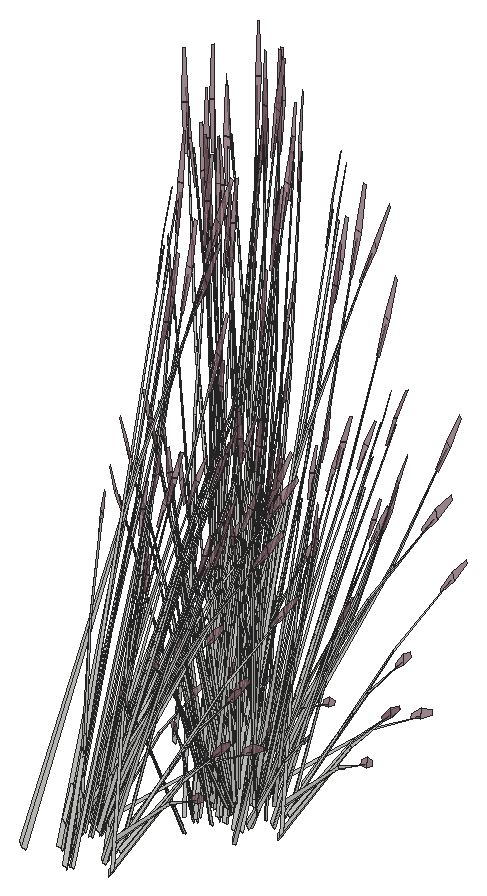
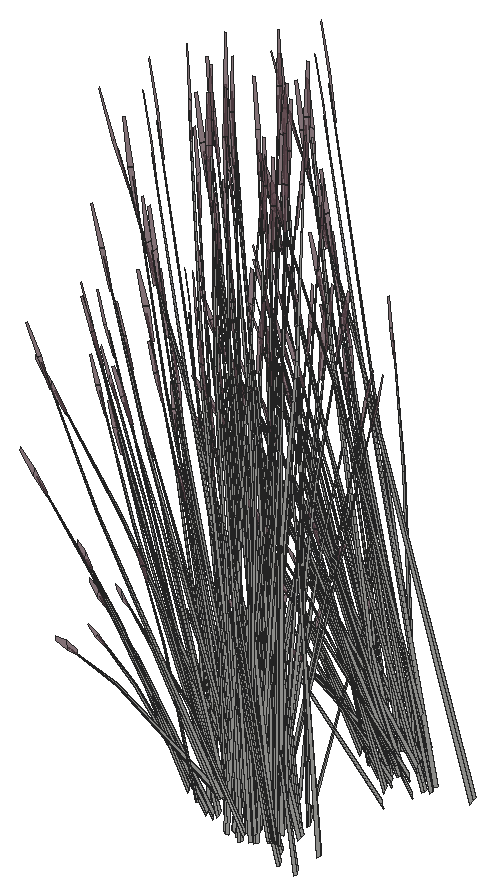
# SketchUp Ruby script. Lengths in inches.
U = 1.inch
M = Sketchup.active_model
def pt(a) = Geom::Point3d.new(a.map { |v| v * U })
def face(e, loops, mat)
  f = e.add_face(loops[0].map { |a| pt(a) })
  loops[1..].each { |l| e.add_face(l.map { |a| pt(a) }).erase! }
  f.material = f.back_material = mat if mat
  f
end
# faces: each face lists its corners as indices into pts; further lists are holes
def faces(e, pts, list, mat = nil) = list.each { |f| face(e, (f[0].is_a?(Array) ? f : [f]).map { |l| l.map { |i| pts[i] } }, mat) }
# xy, xz, yz: faces in a plane at the given z, y or x. An outline is a flat list of corners, or four numbers for a rectangle; further outlines are holes
def ring(l) = l.size == 4 ? [[l[0], l[1]], [l[2], l[1]], [l[2], l[3]], [l[0], l[3]]] : l.each_slice(2).to_a
def flat(e, list, mat, &to3) = list.each { |f| face(e, (f[0].is_a?(Array) ? f : [f]).map { |l| ring(l).map { |u, v| to3.(u, v) } }, mat) }
def xy(e, z, list, mat = nil) = flat(e, list, mat) { |x, y| [x, y, z] }
def xz(e, y, list, mat = nil) = flat(e, list, mat) { |x, z| [x, y, z] }
def yz(e, x, list, mat = nil) = flat(e, list, mat) { |y, z| [x, y, z] }
def lines(e, pts, list) = list.each { |a, b| e.add_line(pt(pts[a]), pt(pts[b])) }
# prism: a flat outline (further loops are holes) pulled along v
def prism(e, loops, v, mat = nil)
  f = face(e, loops, mat); d = Geom::Vector3d.new(v.map { |x| x * U })
  f.pushpull(f.normal.samedirection?(d) ? d.length : -d.length)
end
def box(e, o, s, mat = nil) = prism(e, [[o, [o[0] + s[0], o[1], o[2]], [o[0] + s[0], o[1] + s[1], o[2]], [o[0], o[1] + s[1], o[2]]]], [0, 0, s[2]], mat)
def at(x, y, z, deg = 0) = Geom::Transformation.translation(pt([x, y, z])) * Geom::Transformation.rotation(ORIGIN, Z_AXIS, deg.degrees)
def axes(o, x, y, z) = Geom::Transformation.new([*x, 0, *y, 0, *z, 0, *pt(o).to_a, 1])
def part(name) = M.definitions.add(name)
# library, detail: a bought-in or finely detailed component or shape, given as its bounding box
def library(name, o, s) = part(name).tap { |d| box(d.entities, o, s) }
def detail(e, o, s) = box(e.add_group.entities, o, s)
def put(e, d, t, mat = nil) = e.add_instance(d, t).tap { |i| i.material = mat if mat }
def group(e, t, mat = nil) = e.add_group.tap { |g| g.transformation = t; g.material = mat if mat }.entities
root = M.entities
M.materials.add("LightPink_Translucent").color = [144, 107, 117]
M.materials["LightPink_Translucent"].alpha = 0.75
c1 = part("blade")
p = [[2.15,0.21,22],[0,0.17,0],[0.09,0.45,0],[2.18,0.31,22],[2.29,0.31,22],[0.38,0.45,0],
  [2.48,0.24,33],[2.49,0.24,33],[2.48,0.22,33]]
faces(c1.entities,p,[[0,1,2,3],[4,5,2,3],[6,3,4,7],[8,0,3,6]])
c2 = part("seeds")
p = [[0.3,-0.1,1.38],[-0.01,-0.03,1.59],[-0.01,-0.03,0.03],[0.14,-0.07,-0.07],[0.29,-0.03,3],[0.15,0.01,3.11]]
faces(c2.entities,p,[[0,1,2,3],[1,0,4,5]],"LightPink_Translucent")
c3 = part("blade with seeds")
put(c3.entities,c1,at(0,0,0))
put(c3.entities,c2,axes([2.4,0.25,30.99],[1.5799,-0.05474,1.17369],[-0.12525,1.92788,0.29478],[-0.07173,-0.02425,1.56792]))
put(root,c3,axes([292.33,434.46,4.53],[0.77872,-0.09325,-0.35414],[0.20563,0.53305,0.4572],[0.22316,-0.14318,0.87481]))
put(root,c3,axes([291.69,434.78,5.05],[-0.77872,0.09325,0.35414],[-0.20563,-0.53305,-0.4572],[0.22316,-0.14318,0.87481]))
put(root,c3,axes([292.4,434.69,4.73],[0.61415,0.2744,0.0643],[-0.35756,0.39076,0.50621],[0.1969,-0.12633,0.77189]))
put(root,c3,axes([292.23,434.58,4.73],[0.22187,0.60049,0.48003],[-0.87033,0.10422,0.3958],[0.25651,-0.14123,0.9933]))
put(root,c3,axes([294.57,435.3,4.72],[0.12414,-0.09938,1.74944],[-0.15889,-0.60963,-0.27667],[0.31148,-0.11559,0.14031]))
put(root,c3,axes([292.13,436.23,5.03],[-0.45012,-0.59081,-0.1216],[0.79888,-0.29033,-0.67495],[0.33665,-0.07795,1.02557]))
put(root,c3,axes([292.09,435.72,4.68],[0.24236,-0.59349,-0.51099],[0.83094,0.20343,-0.3958],[0.33455,-0.05442,0.97773]))
put(root,c3,axes([290.78,433.3,2.375],[0.55932,-0.6538,0],[0.93577,0.36461,-0.51607],[0.21313,0.08304,1.63711]))
put(root,c3,axes([292.98,435.89,1.98],[-0.57619,0.0783,1.41583],[-0.09171,-0.62326,0.08104],[0.40356,-0.09434,0.80566]))
put(root,c3,axes([294.03,435.34,2.26],[-0.55463,-0.41721,-0.06488],[0.60744,-0.38228,-0.29416],[0.17212,-0.02691,0.97024]))
put(root,c3,axes([291.93,435.9375,4.98],[0.78611,-0.28816,-0.71045],[0.4381,0.59317,0.08574],[0.37982,-0.06738,1.00501]))
put(root,c3,axes([291.82,436.05,5.05],[-0.74348,-0.18202,0.35414],[0.21685,-0.53102,-0.4572],[0.29933,-0.04869,0.87481]))
put(root,c3,axes([286.73,434.46,1.59],[-0.88056,0.26122,1.28929],[-0.28027,-0.74951,0.50096],[0.54072,0.01247,1.46642]))
put(root,c3,axes([293.61,435.48,1.49],[-0.04675,-0.09906,1.76342],[0.32428,-0.57943,-0.26939],[0.32711,-0.00833,0.30037]))
put(root,c3,axes([289.01,434.85,2.67],[0.90324,-0.43318,-0.29095],[0.60064,0.61207,-0.50002],[0.22285,0.06216,1.59708]))
put(root,c3,axes([292.6,435.99,4.53],[0.74348,0.18202,-0.35414],[-0.21685,0.53102,0.4572],[0.29933,-0.04869,0.87481]))
put(root,c3,axes([291.29,433.7,2.02],[0.83726,0.32623,-0.49651],[-0.50045,0.58498,0],[0.19069,0.0743,1.57504]))
put(root,c3,axes([290.57,435.33,3.875],[-0.37107,0.01478,1.71376],[0.24616,-0.64047,0.13857],[0.5288,0.03961,0.73262]))
put(root,c3,axes([291.05,433.94,2.03],[0.21015,0.56852,-0.30978],[-0.83462,0.16144,0.30978],[0.16826,0.06556,1.38974]))
put(root,c3,axes([292.49,436.21,4.73],[0.32857,0.44488,0.0643],[-0.59916,0.21775,0.50621],[0.26412,-0.04296,0.77189]))
put(root,c3,axes([292.43,436.06,4.73],[-0.25275,0.59491,0.48003],[-0.83094,-0.20343,0.3958],[0.32677,-0.03575,0.9933]))
put(root,c3,axes([290.06,434.95,2.06],[0.9306,0.10697,-0.62353],[-0.19638,0.65984,-0.16365],[0.27771,0.07995,1.37633]))
put(root,c3,axes([294.18,436.1,2.77],[-0.55274,0.10771,1.1486],[0.26018,-0.44517,0.84392],[0.29323,0.03046,0.25299]))
put(root,c3,axes([293.92,437.98,4.71],[-0.08089,-0.05712,1.77383],[0.17695,-0.61228,-0.16761],[0.31864,-0.03912,0.31391]))
put(root,c3,axes([289.58,435.16,2.21],[0.53742,0.54764,-0.44739],[-0.81403,0.38564,0.21531],[0.17391,0.06776,1.43643]))
put(root,c3,axes([293.22,437.47,3.93],[-0.17122,-0.54847,-0.03492],[0.80929,-0.12609,-0.15832],[0.169,0.03477,0.52218]))
put(root,c3,axes([291.12,437.46,5.03],[0.0479,-0.66354,-0.1216],[0.90696,0.01814,-0.67495],[0.3493,0.04609,1.02557]))
put(root,c3,axes([290.98,437.2,5.05],[-0.50902,-0.40851,0.35414],[0.58122,-0.38671,-0.4572],[0.29531,0.05884,0.87481]))
put(root,c3,axes([293.14,436.8125,2.59],[-0.21545,-0.16047,1.43002],[0.28033,-0.53085,-0.30754],[0.43591,0.07191,0.61141]))
put(root,c3,axes([291.91,437.06,4.72],[0.19191,-0.01103,1.74944],[0.52639,-0.5069,-0.27667],[0.34136,0.06691,0.14031]))
put(root,c3,axes([291.16,437.14,4.98],[0.89428,0.01571,-0.71045],[-0.06006,0.66153,0.08574],[0.37886,0.06981,1.00501]))
put(root,c3,axes([292.625,435.79,2.375],[1.11865,0,0],[0,0.72922,-0.51607],[0,0.16609,1.63711]))
put(root,c3,axes([291.7,437.41,4.53],[0.50902,0.40851,-0.35414],[-0.58122,0.38671,0.4572],[0.29531,0.05884,0.87481]))
put(root,c3,axes([291.44,437.57,4.73],[-0.04505,0.49615,0.0643],[-0.68022,-0.0136,0.50621],[0.26056,0.05192,0.77189]))
put(root,c3,axes([291.5,437.41,4.73],[-0.65964,0.42992,0.48003],[-0.5689,-0.45657,0.3958],[0.30948,0.0793,0.9933]))
put(root,c3,axes([296.18,444.44,2.59],[-0.25429,0.13207,1.43002],[-0.76157,-0.23115,-0.30754],[0.14117,-0.28747,0.61141]))
put(root,c3,axes([294.29,443.73,1.49],[-0.15005,0.02351,1.76342],[-0.82981,-0.26461,-0.26939],[0.01392,-0.22072,0.30037]))
put(root,c3,axes([296.8,445.42,4.98],[0.02328,-0.60353,-0.71045],[0.98022,0.04053,0.08574],[0.10344,-0.25568,1.00501]))
put(root,c3,axes([289.87,436.36,3.875],[-0.3323,-0.11241,1.71376],[0.68769,-0.4716,0.13857],[0.42861,0.21275,0.73262]))
put(root,c3,axes([289.9375,434.88,4.47],[-0.77304,-0.33901,1.38283],[0.81626,-0.52782,0.59665],[0.24941,0.31809,1.33663]))
put(root,c3,axes([298.17,444.48,4.72],[-0.00864,-0.12985,1.74944],[-0.72937,-0.3753,-0.27667],[0.11277,-0.2275,0.14031]))
put(root,c3,axes([295.1,444.45,4.53],[0.2697,-0.50175,-0.35414],[0.78684,0.14635,0.4572],[-0.07215,-0.20201,0.87481]))
put(root,c3,axes([295.7,445.12,3.875],[-0.16657,0.22426,1.71376],[-0.69879,-0.4641,0.13857],[0.31524,-0.28926,0.73262]))
put(root,c3,axes([297.97,444.01,4.71],[-0.09085,0.04984,1.77383],[-0.89014,-0.16814,-0.16761],[-0.03222,-0.21748,0.31391]))
put(root,c3,axes([291.1,437.64,2.77],[-0.5037,-0.18761,1.1486],[0.6504,-0.19062,0.84392],[0.17543,0.16147,0.25299]))
put(root,c3,axes([289.33,438.18,5.03],[0.53309,-0.55848,-0.1216],[0.77201,0.32175,-0.67495],[0.26836,0.15779,1.02557]))
put(root,c3,axes([295.25,443.39,2.77],[0.11476,0.38047,1.1486],[-0.63664,-0.21072,0.84392],[0.06851,-0.19481,0.25299]))
put(root,c3,axes([296.6,445.22,4.68],[-0.64041,-0.4384,-0.51099],[0.67652,-0.38394,-0.3958],[0.09744,-0.22274,0.97773]))
put(root,c3,axes([288.64,438.64,4.71],[0.00265,-0.07899,1.77383],[0.76665,-0.34851,-0.16761],[0.2663,0.12439,0.31391]))
put(root,c3,axes([291.24,438.34,1.49],[0.06518,-0.0942,1.76342],[0.82057,-0.27742,-0.26939],[0.24877,0.14358,0.30037]))
put(root,c3,axes([289.96,437.9,4.68],[0.88277,-0.1551,-0.51099],[0.15442,0.58737,-0.3958],[0.23711,0.16832,0.97773]))
put(root,c3,axes([295.2,444.57,4.73],[0.88151,0.17057,0.48003],[-0.30143,0.56078,0.3958],[-0.05297,-0.22053,0.9933]))
put(root,c3,axes([297.27,445.45,5.03],[-0.98321,-0.03233,-0.1216],[0.02687,-0.61208,-0.67495],[0.0683,-0.23574,1.02557]))
put(root,c3,axes([297.21,445.06,4.53],[0.60531,-0.34352,-0.35414],[0.573,0.39225,0.4572],[0.08718,-0.19929,0.87481]))
put(root,c3,axes([295.4375,444.53,4.73],[0.6592,-0.22175,0.0643],[0.32265,0.40436,0.50621],[-0.06366,-0.17825,0.77189]))
put(root,c3,axes([291.18,438.5,2.67],[-0.57368,-0.02046,1.0506],[0.37886,-0.43461,0.58006],[0.22663,0.15441,0.8241]))
put(root,c3,axes([289.31,437.44,2.59],[0.01579,-0.21629,1.43002],[0.75442,-0.24159,-0.30754],[0.23289,0.25887,0.61141]))
put(root,c3,axes([297.96,444.85,1.49],[-0.1339,-0.0514,1.76342],[-0.34394,-0.57425,-0.26939],[0.23202,-0.15583,0.30037]))
put(root,c3,axes([295.19,444.98,5.05],[-0.2697,0.50175,0.35414],[-0.78684,-0.14635,-0.4572],[-0.07215,-0.20201,0.87481]))
put(root,c3,axes([297.2,445.19,4.73],[0.63704,0.44518,0.48003],[-0.67652,0.38394,0.3958],[0.11751,-0.20886,0.9933]))
put(root,c3,axes([297.4375,445.23,4.73],[0.73517,0.0304,0.0643],[-0.02016,0.45906,0.50621],[0.07693,-0.17585,0.77189]))
put(root,c3,axes([296.89,445.55,5.05],[-0.60531,0.34352,0.35414],[-0.573,-0.39225,-0.4572],[0.08718,-0.19929,0.87481]))
put(root,c3,axes([297.96,446.47,4.98],[0.4673,-0.51481,-0.71045],[0.81887,0.36587,0.08574],[0.27902,-0.18652,1.00501]))
put(root,c3,axes([292.9,444.97,2.375],[-0.55932,-0.6538,0],[0.93577,-0.36461,-0.51607],[0.21313,-0.08304,1.63711]))
put(root,c3,axes([297.93,446.23,4.68],[-0.22982,-0.59576,-0.51099],[0.87033,-0.10422,-0.3958],[0.24941,-0.16002,0.97773]))
put(root,c3,axes([298.34,446.66,5.03],[-0.82753,-0.35977,-0.1216],[0.47675,-0.52101,-0.67495],[0.2338,-0.18111,1.02557]))
put(root,c3,axes([293.66,444.87,2.02],[0.83726,-0.32623,-0.49651],[0.50045,0.58498,0],[0.19069,-0.0743,1.57504]))
put(root,c3,axes([298.63,446,2.59],[-0.31959,-0.01933,1.43002],[-0.32741,-0.51843,-0.30754],[0.39262,-0.14666,0.61141]))
put(root,c3,axes([300.38,446.5,4.71],[-0.11685,-0.00496,1.77383],[-0.48522,-0.53096,-0.16761],[0.19486,-0.17458,0.31391]))
put(root,c3,axes([294.66,446.21,2.06],[0.60257,-0.49041,-0.62353],[0.74854,0.44469,-0.16365],[0.24146,-0.12234,1.37633]))
put(root,c3,axes([299,445.04,2.77],[-0.29798,0.33213,1.1486],[-0.25612,-0.44624,0.84392],[0.24611,-0.11182,0.25299]))
put(root,c3,axes([298.58,446.29,4.53],[0.77872,-0.09325,-0.35414],[0.20563,0.53305,0.4572],[0.22316,-0.14318,0.87481]))
put(root,c3,axes([293.61,447.07,2.21],[0.43405,-0.58792,-0.44739],[0.90188,0.28295,0.21531],[0,-0.13553,1.43643]))
put(root,c3,axes([294,446.78,2.67],[-0.10425,-0.7445,-0.29095],[1.08575,-0.04502,-0.50002],[0.19119,-0.09917,1.59708]))
put(root,c3,axes([297.94,446.61,5.05],[-0.77872,0.09325,0.35414],[-0.20563,-0.53305,-0.4572],[0.22316,-0.14318,0.87481]))
put(root,c3,axes([293.86,445.13,2.03],[0.83462,0.16144,-0.30978],[-0.21015,0.56852,0.30978],[0.16826,-0.06556,1.38974]))
put(root,c3,axes([298.65,446.52,4.73],[0.61415,0.2744,0.0643],[-0.35756,0.39076,0.50621],[0.1969,-0.12633,0.77189]))
put(root,c3,axes([298.47,446.41,4.73],[0.22187,0.60049,0.48003],[-0.87033,0.10422,0.3958],[0.25651,-0.14123,0.9933]))
put(root,c3,axes([300.82,447.13,4.72],[0.12414,-0.09938,1.74944],[-0.15889,-0.60963,-0.27667],[0.31148,-0.11559,0.14031]))
put(root,c3,axes([294.15,447.36,2.43],[1.00799,0.31623,0.24065],[-0.48511,0.65709,0.50002],[0,-0.15147,1.60543]))
put(root,c3,axes([288.01,450.35,3.875],[-0.16657,0.22426,1.71376],[-0.69879,-0.4641,0.13857],[0.31524,-0.28926,0.73262]))
put(root,c3,axes([293.82,446.92,2.72],[-0.97146,0.04028,0.44739],[-0.08785,-0.66859,-0.21531],[0.17391,-0.06776,1.43643]))
put(root,c3,axes([298.38,448.06,5.03],[-0.45012,-0.59081,-0.1216],[0.79888,-0.29033,-0.67495],[0.33665,-0.07795,1.02557]))
put(root,c3,axes([298.34,447.55,4.68],[0.24236,-0.59349,-0.51099],[0.83094,0.20343,-0.3958],[0.33455,-0.05442,0.97773]))
put(root,c3,axes([297.02,445.14,2.375],[0.55932,-0.6538,0],[0.93577,0.36461,-0.51607],[0.21313,0.08304,1.63711]))
put(root,c3,axes([293.79,447.16,2.36],[0.38895,0.72959,0.45755],[-1.11135,0.2537,0.17955],[0.01358,-0.13406,1.58856]))
put(root,c3,axes([299.23,447.72,1.98],[-0.57619,0.0783,1.41583],[-0.09171,-0.62326,0.08104],[0.40356,-0.09434,0.80566]))
put(root,c3,axes([300.27,447.17,2.26],[-0.55463,-0.41721,-0.06488],[0.60744,-0.38228,-0.29416],[0.17212,-0.02691,0.97024]))
put(root,c3,axes([295.1875,447.22,2.21],[0,-0.75495,0],[1.11865,0,0],[0,0,1.79456]))
put(root,c3,axes([296.54,445.48,2.48],[-0.83726,-0.32623,0.49651],[0.50045,-0.58498,0],[0.19069,0.0743,1.57504]))
put(root,c3,axes([298.18,447.77,4.98],[0.78611,-0.28816,-0.71045],[0.4381,0.59317,0.08574],[0.37982,-0.06738,1.00501]))
put(root,c3,axes([294.66,446.75,2.36],[-0.74176,0.59212,0.45755],[-0.88124,-0.52269,0.17955],[0.17882,-0.05909,1.58856]))
put(root,c3,axes([295.47,447.81,2.3],[-0.83213,-0.56158,-0.06131],[0.83263,-0.56193,0],[-0.02906,-0.01961,1.75571]))
put(root,c3,axes([293.37,445.77,2.47],[-0.25843,0.64844,0.17642],[-0.9457,-0.1835,0.35086],[0.16336,-0.00316,1.60407]))
put(root,c3,axes([298.0625,447.88,5.05],[-0.74348,-0.18202,0.35414],[0.21685,-0.53102,-0.4572],[0.29933,-0.04869,0.87481]))
put(root,c3,axes([292.98,446.29,1.59],[-0.88056,0.26122,1.28929],[-0.28027,-0.74951,0.50096],[0.54072,0.01247,1.46642]))
put(root,c3,axes([295.34,446.49,2.62],[0.17258,-0.58229,0.1448],[0.84319,0.10108,-0.41347],[0.15345,0.05979,1.26744]))
put(root,c3,axes([299.85,447.3125,1.49],[-0.04675,-0.09906,1.76342],[0.32428,-0.57943,-0.26939],[0.32711,-0.00833,0.30037]))
put(root,c3,axes([294.98,446.65,2.72],[-0.53742,-0.54764,0.44739],[0.81403,-0.38564,-0.21531],[0.17391,0.06776,1.43643]))
put(root,c3,axes([290.27,450.09,1.49],[-0.1339,-0.0514,1.76342],[-0.34394,-0.57425,-0.26939],[0.23202,-0.15583,0.30037]))
put(root,c3,axes([295.26,446.68,2.67],[0.90324,-0.43318,-0.29095],[0.60064,0.61207,-0.50002],[0.22285,0.06216,1.59708]))
put(root,c3,axes([298.85,447.82,4.53],[0.74348,0.18202,-0.35414],[-0.21685,0.53102,0.4572],[0.29933,-0.04869,0.87481]))
put(root,c3,axes([297.53,445.53,2.02],[0.83726,0.32623,-0.49651],[-0.50045,0.58498,0],[0.19069,0.0743,1.57504]))
put(root,c3,axes([295.94,447.39,2.21],[1.00089,0,0],[0,0.67548,0],[0,0,1.78407]))
put(root,c3,axes([296.23,445.81,2.47],[-0.96132,0.17317,0.17642],[-0.23737,-0.64447,0.35086],[0.08574,0.0939,1.60407]))
put(root,c3,axes([290.27,451.7,4.98],[0.4673,-0.51481,-0.71045],[0.81887,0.36587,0.08574],[0.27902,-0.18652,1.00501]))
put(root,c3,axes([290.24,451.46,4.68],[-0.22982,-0.59576,-0.51099],[0.87033,-0.10422,-0.3958],[0.24941,-0.16002,0.97773]))
put(root,c3,axes([296.82,447.17,3.875],[-0.37107,0.01478,1.71376],[0.24616,-0.64047,0.13857],[0.5288,0.03961,0.73262]))
put(root,c3,axes([297.3,445.77,2.03],[0.21015,0.56852,-0.30978],[-0.83462,0.16144,0.30978],[0.16826,0.06556,1.38974]))
put(root,c3,axes([298.74,448.05,4.73],[0.32857,0.44488,0.0643],[-0.59916,0.21775,0.50621],[0.26412,-0.04296,0.77189]))
put(root,c3,axes([290.65,451.89,5.03],[-0.82753,-0.35977,-0.1216],[0.47675,-0.52101,-0.67495],[0.2338,-0.18111,1.02557]))
put(root,c3,axes([295.62,447.05,2.38],[-1.13071,-0.13747,0.49198],[0.23011,-0.77639,0.19306],[0.16524,0.07497,1.70813]))
put(root,c3,axes([298.67,447.89,4.73],[-0.25275,0.59491,0.48003],[-0.83094,-0.20343,0.3958],[0.32677,-0.03575,0.9933]))
put(root,c3,axes([294.72,448.96,2.2],[-0.29189,-0.56252,0],[0.83351,-0.19699,0],[0,0,1.54371]))
put(root,c3,axes([295.8125,448.88,2.18],[0.93921,-0.22138,-0.19198],[0.33003,0.6377,0.00008],[0.10367,-0.02447,1.73897]))
put(root,c3,axes([296.14,449.15,2.47],[0.25843,-0.64844,0.17642],[0.9457,0.1835,0.35086],[-0.16336,0.00316,1.60407]))
put(root,c3,axes([295.92,447.68,2.21],[0.62448,0.42144,0],[-0.62448,0.42144,0],[0,0,1.69266]))
put(root,c3,axes([290.94,451.23,2.59],[-0.31959,-0.01933,1.43002],[-0.32741,-0.51843,-0.30754],[0.39262,-0.14666,0.61141]))
put(root,c3,axes([292.69,451.73,4.71],[-0.11685,-0.00496,1.77383],[-0.48522,-0.53096,-0.16761],[0.19486,-0.17458,0.31391]))
put(root,c3,axes([297.61,447.5,2.47],[-0.70288,-0.47526,0.17642],[0.70832,-0.46097,0.35086],[-0.07763,0.09706,1.60407]))
put(root,c3,axes([296.3125,446.78,2.06],[0.9306,0.10697,-0.62353],[-0.19638,0.65984,-0.16365],[0.27771,0.07995,1.37633]))
put(root,c3,axes([300.42,447.93,2.77],[-0.55274,0.10771,1.1486],[0.26018,-0.44517,0.84392],[0.29323,0.03046,0.25299]))
put(root,c3,axes([291.3125,450.28,2.77],[-0.29798,0.33213,1.1486],[-0.25612,-0.44624,0.84392],[0.24611,-0.11182,0.25299]))
put(root,c3,axes([294.51,449.22,2.2],[-0.90188,-0.29293,0],[0.43405,-0.60866,0],[0,0,1.62707]))
put(root,c3,axes([295.91,447.1875,2.72],[0.43405,-0.58792,0.44739],[0.90188,0.28295,-0.21531],[0,0.13553,1.43643]))
put(root,c3,axes([300.17,449.81,4.71],[-0.08089,-0.05712,1.77383],[0.17695,-0.61228,-0.16761],[0.31864,-0.03912,0.31391]))
put(root,c3,axes([290.88,451.53,4.53],[0.77872,-0.09325,-0.35414],[0.20563,0.53305,0.4572],[0.22316,-0.14318,0.87481]))
put(root,c3,axes([295.75,447.52,2.29],[0,0.75458,-0.05637],[-1.11865,0,0],[0,0.02371,1.79368]))
put(root,c3,axes([295.83,446.99,2.21],[0.53742,0.54764,-0.44739],[-0.81403,0.38564,0.21531],[0.17391,0.06776,1.43643]))
put(root,c3,axes([299.46,449.3,3.93],[-0.17122,-0.54847,-0.03492],[0.80929,-0.12609,-0.15832],[0.169,0.03477,0.52218]))
put(root,c3,axes([297.37,449.29,5.03],[0.0479,-0.66354,-0.1216],[0.90696,0.01814,-0.67495],[0.3493,0.04609,1.02557]))
put(root,c3,axes([298.19,447.51,2.48],[0,-0.65246,0.49651],[1.00089,0,0],[0,0.1486,1.57504]))
put(root,c3,axes([295.68,448,2.72],[0.97146,-0.04028,0.44739],[0.08785,0.66859,-0.21531],[-0.17391,0.06776,1.43643]))
put(root,c3,axes([296.29,447.32,2.62],[0.83351,-0.19028,0.1448],[0.29189,0.54335,-0.41347],[0,0.11958,1.26744]))
put(root,c3,axes([297.23,449.03,5.05],[-0.50902,-0.40851,0.35414],[0.58122,-0.38671,-0.4572],[0.29531,0.05884,0.87481]))
put(root,c3,axes([299.39,448.65,2.59],[-0.21545,-0.16047,1.43002],[0.28033,-0.53085,-0.30754],[0.43591,0.07191,0.61141]))
put(root,c3,axes([295.54,449.23,2.2],[0.90188,0.29293,0],[-0.43405,0.60866,0],[0,0,1.74954]))
put(root,c3,axes([290.96,451.76,4.73],[0.61415,0.2744,0.0643],[-0.35756,0.39076,0.50621],[0.1969,-0.12633,0.77189]))
put(root,c3,axes([290.78,451.64,4.73],[0.22187,0.60049,0.48003],[-0.87033,0.10422,0.3958],[0.25651,-0.14123,0.9933]))
put(root,c3,axes([298.15,448.89,4.72],[0.19191,-0.01103,1.74944],[0.52639,-0.5069,-0.27667],[0.34136,0.06691,0.14031]))
put(root,c3,axes([293.13,452.37,4.72],[0.12414,-0.09938,1.74944],[-0.15889,-0.60963,-0.27667],[0.31148,-0.11559,0.14031]))
put(root,c3,axes([295.7,448.29,2.62],[0.66093,0.39201,0.1448],[-0.5513,0.44227,-0.41347],[-0.15345,0.05979,1.26744]))
put(root,c3,axes([297.41,448.97,4.98],[0.89428,0.01571,-0.71045],[-0.06006,0.66153,0.08574],[0.37886,0.06981,1.00501]))
put(root,c3,axes([296.4,449.5,2.48],[0.83726,-0.32623,0.49651],[0.50045,0.58498,0],[-0.19069,0.0743,1.57504]))
put(root,c3,axes([295.21,448.98,2.29],[0.38895,0.74956,-0.06012],[-1.11135,0.26265,0],[0.01358,0.02618,1.72173]))
